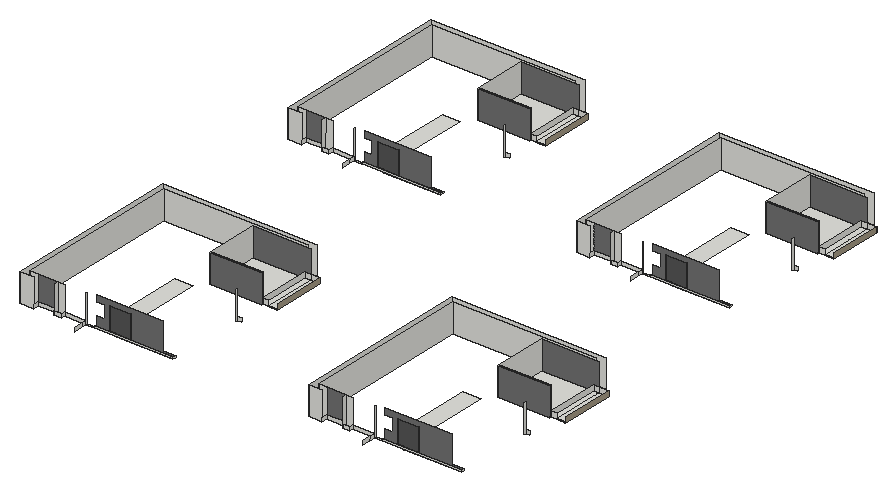
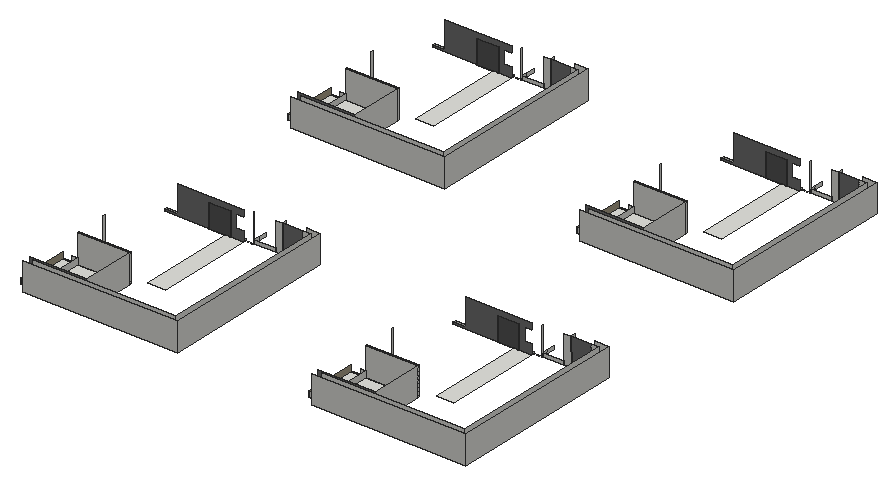
# SketchUp Ruby script. Lengths in inches.
U = 1.inch
M = Sketchup.active_model
def pt(a) = Geom::Point3d.new(a.map { |v| v * U })
def face(e, loops, mat)
  f = e.add_face(loops[0].map { |a| pt(a) })
  loops[1..].each { |l| e.add_face(l.map { |a| pt(a) }).erase! }
  f.material = f.back_material = mat if mat
  f
end
# faces: each face lists its corners as indices into pts; further lists are holes
def faces(e, pts, list, mat = nil) = list.each { |f| face(e, (f[0].is_a?(Array) ? f : [f]).map { |l| l.map { |i| pts[i] } }, mat) }
# xy, xz, yz: faces in a plane at the given z, y or x. An outline is a flat list of corners, or four numbers for a rectangle; further outlines are holes
def ring(l) = l.size == 4 ? [[l[0], l[1]], [l[2], l[1]], [l[2], l[3]], [l[0], l[3]]] : l.each_slice(2).to_a
def flat(e, list, mat, &to3) = list.each { |f| face(e, (f[0].is_a?(Array) ? f : [f]).map { |l| ring(l).map { |u, v| to3.(u, v) } }, mat) }
def xy(e, z, list, mat = nil) = flat(e, list, mat) { |x, y| [x, y, z] }
def xz(e, y, list, mat = nil) = flat(e, list, mat) { |x, z| [x, y, z] }
def yz(e, x, list, mat = nil) = flat(e, list, mat) { |y, z| [x, y, z] }
def lines(e, pts, list) = list.each { |a, b| e.add_line(pt(pts[a]), pt(pts[b])) }
# prism: a flat outline (further loops are holes) pulled along v
def prism(e, loops, v, mat = nil)
  f = face(e, loops, mat); d = Geom::Vector3d.new(v.map { |x| x * U })
  f.pushpull(f.normal.samedirection?(d) ? d.length : -d.length)
end
def box(e, o, s, mat = nil) = prism(e, [[o, [o[0] + s[0], o[1], o[2]], [o[0] + s[0], o[1] + s[1], o[2]], [o[0], o[1] + s[1], o[2]]]], [0, 0, s[2]], mat)
def at(x, y, z, deg = 0) = Geom::Transformation.translation(pt([x, y, z])) * Geom::Transformation.rotation(ORIGIN, Z_AXIS, deg.degrees)
def axes(o, x, y, z) = Geom::Transformation.new([*x, 0, *y, 0, *z, 0, *pt(o).to_a, 1])
def part(name) = M.definitions.add(name)
# library, detail: a bought-in or finely detailed component or shape, given as its bounding box
def library(name, o, s) = part(name).tap { |d| box(d.entities, o, s) }
def detail(e, o, s) = box(e.add_group.entities, o, s)
def put(e, d, t, mat = nil) = e.add_instance(d, t).tap { |i| i.material = mat if mat }
def group(e, t, mat = nil) = e.add_group.tap { |g| g.transformation = t; g.material = mat if mat }.entities
root = M.entities
M.materials.add("[Color M05]").color = [114, 114, 114]
M.materials.add("[Color M06]").color = [86, 86, 86]
M.materials.add("[Concrete Tile]").color = [165, 155, 133]
M.materials.add("[Granite Brown]").color = [89, 59, 61]
xy(root,510,[[523.04,1822.9375,557.4,1827.4375],[648.79,1822.9375,650.48,1827.4375],[650.48,1822.9375,890.875,1822.9375,890.875,1835.1875,701.59,1835.1875,701.59,1837.0625,650.48,1837.0625],[1741.23,1822.9375,1775.59,1827.4375],[1866.98,1822.9375,1868.66,1827.4375],
  [1868.66,1822.9375,2109.0625,1822.9375,2109.0625,1835.1875,1919.77,1835.1875,1919.77,1837.0625,1868.66,1837.0625],[557.88,1827.4375,632.49,1829.625],[632.49,1827.4375,648.79,1837.0625],[648.79,1827.4375,650.48,1837.0625],[1776.07,1827.4375,1850.67,1829.625],
  [1850.67,1827.4375,1866.98,1837.0625],[1866.98,1827.4375,1868.66,1837.0625],[557.88,1829.625,632.49,1835.1875],[1776.07,1829.625,1850.67,1835.1875],[557.4,1835.1875,632.49,2246.6875],
  [1775.59,1835.1875,1850.67,2246.6875],[671.875,2290,890.875,2295.875],[1890.0625,2290,2109.0625,2295.875],[671.875,2295.875,890.875,2518.89],[890.875,2295.875,913.875,2518.89],
  [913.875,2295.875,954.6875,2518.89],[1890.0625,2295.875,2109.0625,2518.89],[2109.0625,2295.875,2132.0625,2518.89],[2132.0625,2295.875,2172.875,2518.89],[523.04,3237.625,557.4,3242.125],
  [648.79,3237.625,650.48,3242.125],[650.48,3237.625,890.875,3237.625,890.875,3249.875,701.59,3249.875,701.59,3251.75,650.48,3251.75],[1741.23,3237.625,1775.59,3242.125],[1866.98,3237.625,1868.66,3242.125],[1868.66,3237.625,2109.0625,3237.625,2109.0625,3249.875,1919.77,3249.875,1919.77,3251.75,1868.66,3251.75],
  [557.88,3242.125,632.49,3244.3125],[632.49,3242.125,648.79,3251.75],[648.79,3242.125,650.48,3251.75],[1776.07,3242.125,1850.67,3244.3125],[1850.67,3242.125,1866.98,3251.75],
  [1866.98,3242.125,1868.66,3251.75],[557.88,3244.3125,632.49,3249.875],[1776.07,3244.3125,1850.67,3249.875],[557.4,3249.875,632.49,3661.375],[1775.59,3249.875,1850.67,3661.375],
  [671.875,3704.6875,890.875,3710.5625],[1890.0625,3704.6875,2109.0625,3710.5625],[671.875,3710.5625,890.875,3933.57],[890.875,3710.5625,913.875,3933.57],[913.875,3710.5625,954.6875,3933.57],
  [1890.0625,3710.5625,2109.0625,3933.57],[2109.0625,3710.5625,2132.0625,3933.57],[2132.0625,3710.5625,2172.875,3933.57]])
xy(root,510,[[557.4,1822.9375,557.88,1827.4375],[1775.59,1822.9375,1776.07,1827.4375],[557.4,1827.4375,557.88,1829.625],[1775.59,1827.4375,1776.07,1829.625],[557.4,1829.625,557.88,1835.1875],
  [1775.59,1829.625,1776.07,1835.1875],[557.4,3237.625,557.88,3242.125],[1775.59,3237.625,1776.07,3242.125],[557.4,3242.125,557.88,3244.3125],[1775.59,3242.125,1776.07,3244.3125],
  [557.4,3244.3125,557.88,3249.875],[1775.59,3244.3125,1776.07,3249.875]],"[Granite Brown]")
xy(root,510.3125,[[611.65,1835.1875,632.49,1837.0625],[1829.84,1835.1875,1850.67,1837.0625],[611.65,3249.875,632.49,3251.75],[1829.84,3249.875,1850.67,3251.75]])
xz(root,1799.9375,[[262.875,510,319.53,630],[1481.0625,510,1537.72,630]])
xz(root,1806.5625,[[401.17,510,401.17,525.4375,401.25,525.4375],[401.17,510,431.33,510,431.33,525.4375,401.25,525.4375],[1619.36,510,1619.36,525.4375,1619.4375,525.4375],[1619.36,510,1649.52,510,1649.52,525.4375,1619.4375,525.4375]])
xz(root,1822.9375,[[285.875,510,319.53,630],[319.53,510,401.17,525.4375],[401.17,510,401.77,630,431.33,630,431.33,510],[431.33,510,523.04,525.4375],[557.88,510,890.875,516.375],
  [1504.0625,510,1537.72,630],[1537.72,510,1619.36,525.4375],[1619.36,510,1619.96,630,1649.52,630,1649.52,510],[1649.52,510,1741.23,525.4375],[1776.07,510,2109.0625,516.375]])
xz(root,1822.9375,[[401.17,510,401.77,630,319.53,630,319.53,525.4375,401.17,525.4375],[1619.36,510,1619.96,630,1537.72,630,1537.72,525.4375,1619.36,525.4375]],"[Color M05]")
xz(root,1835.1875,[[611.65,509.5625,632.49,510],[1829.84,509.5625,1850.67,510],[611.65,510,632.49,510.3125],[1829.84,510,1850.67,510.3125]])
xz(root,1835.1875,[[557.88,510,611.65,510,611.65,608.125,701.59,608.125,701.59,510,890.875,510,890.875,517.25,838.125,517.25,838.125,630,557.88,630,557.88,603.53,589.71,603.53,589.71,551.24,557.88,551.24],[1776.07,510,1829.84,510,1829.84,608.125,1919.77,608.125,1919.77,510,2109.0625,510,2109.0625,517.25,2056.3125,517.25,2056.3125,630,1776.07,630,1776.07,603.53,1807.9,603.53,1807.9,551.24,1776.07,551.24]],"[Color M05]")
xz(root,1837.0625,[[632.49,510,701.59,510,701.59,608.125,611.65,608.125,611.65,510.3125,632.49,510.3125],[1850.67,510,1919.77,510,1919.77,608.125,1829.84,608.125,1829.84,510.3125,1850.67,510.3125]],"[Color M06]")
xz(root,2156.01,[[894.3125,510,913.875,527.36],[2112.5,510,2132.0625,527.36]])
xz(root,2290,[[671.875,510,890.875,630],[1890.0625,510,2109.0625,630]],"[Color M05]")
xz(root,2295.875,[[671.875,510,890.875,630],[890.875,510,913.875,534.0625],[913.875,510,930.75,511.75],[930.75,510,954.6875,511.75],[1890.0625,510,2109.0625,630],
  [2109.0625,510,2132.0625,534.0625],[2132.0625,510,2148.9375,511.75],[2148.9375,510,2172.875,511.75]])
xz(root,2518.89,[[890.875,510,913.875,534.0625],[913.875,510,954.6875,534.0625],[2109.0625,510,2132.0625,534.0625],[2132.0625,510,2172.875,534.0625]])
xz(root,2518.89,[[671.875,510,890.875,510,890.875,534.0625,913.875,534.0625,913.875,630,671.875,630],[1890.0625,510,2109.0625,510,2109.0625,534.0625,2132.0625,534.0625,2132.0625,630,1890.0625,630]],"[Color M05]")
xz(root,2531.375,[[285.875,510,890.875,630],[1504.0625,510,2109.0625,630]])
xz(root,2554.375,[[262.875,510,913.875,630],[1481.0625,510,2132.0625,630]])
xz(root,3214.625,[[262.875,510,319.53,630],[1481.0625,510,1537.72,630]])
xz(root,3221.25,[[401.17,510,401.17,525.4375,401.25,525.4375],[401.17,510,431.33,510,431.33,525.4375,401.25,525.4375],[1619.36,510,1619.36,525.4375,1619.4375,525.4375],[1619.36,510,1649.52,510,1649.52,525.4375,1619.4375,525.4375]])
xz(root,3237.625,[[285.875,510,319.53,630],[319.53,510,401.17,525.4375],[401.17,510,401.77,630,431.33,630,431.33,510],[431.33,510,523.04,525.4375],[557.88,510,890.875,516.375],
  [1504.0625,510,1537.72,630],[1537.72,510,1619.36,525.4375],[1619.36,510,1619.96,630,1649.52,630,1649.52,510],[1649.52,510,1741.23,525.4375],[1776.07,510,2109.0625,516.375]])
xz(root,3237.625,[[401.17,510,401.77,630,319.53,630,319.53,525.4375,401.17,525.4375],[1619.36,510,1619.96,630,1537.72,630,1537.72,525.4375,1619.36,525.4375]],"[Color M05]")
xz(root,3249.875,[[611.65,509.5625,632.49,510],[1829.84,509.5625,1850.67,510],[611.65,510,632.49,510.3125],[1829.84,510,1850.67,510.3125]])
xz(root,3249.875,[[557.88,510,611.65,510,611.65,608.125,701.59,608.125,701.59,510,890.875,510,890.875,517.25,838.125,517.25,838.125,630,557.88,630,557.88,603.53,589.71,603.53,589.71,551.24,557.88,551.24],[1776.07,510,1829.84,510,1829.84,608.125,1919.77,608.125,1919.77,510,2109.0625,510,2109.0625,517.25,2056.3125,517.25,2056.3125,630,1776.07,630,1776.07,603.53,1807.9,603.53,1807.9,551.24,1776.07,551.24]],"[Color M05]")
xz(root,3251.75,[[632.49,510,701.59,510,701.59,608.125,611.65,608.125,611.65,510.3125,632.49,510.3125],[1850.67,510,1919.77,510,1919.77,608.125,1829.84,608.125,1829.84,510.3125,1850.67,510.3125]],"[Color M06]")
xz(root,3570.7,[[894.3125,510,913.875,527.36],[2112.5,510,2132.0625,527.36]])
xz(root,3704.6875,[[671.875,510,890.875,630],[1890.0625,510,2109.0625,630]],"[Color M05]")
xz(root,3710.5625,[[671.875,510,890.875,630],[890.875,510,913.875,534.0625],[913.875,510,930.75,511.75],[930.75,510,954.6875,511.75],[1890.0625,510,2109.0625,630],
  [2109.0625,510,2132.0625,534.0625],[2132.0625,510,2148.9375,511.75],[2148.9375,510,2172.875,511.75]])
xz(root,3933.57,[[890.875,510,913.875,534.0625],[913.875,510,954.6875,534.0625],[2109.0625,510,2132.0625,534.0625],[2132.0625,510,2172.875,534.0625]])
xz(root,3933.57,[[671.875,510,890.875,510,890.875,534.0625,913.875,534.0625,913.875,630,671.875,630],[1890.0625,510,2109.0625,510,2109.0625,534.0625,2132.0625,534.0625,2132.0625,630,1890.0625,630]],"[Color M05]")
xz(root,3946.0625,[[285.875,510,890.875,630],[1504.0625,510,2109.0625,630]])
xz(root,3969.0625,[[262.875,510,913.875,630],[1481.0625,510,2132.0625,630]])
yz(root,262.875,[[1799.9375,510,2554.375,630],[3214.625,510,3969.0625,630]])
yz(root,285.875,[[1822.9375,510,2531.375,630],[3237.625,510,3946.0625,630]])
yz(root,319.53,[[1799.9375,510,1822.9375,525.4375],[3214.625,510,3237.625,525.4375]])
yz(root,401.17,[[1806.5625,510,1822.9375,525.4375],[3221.25,510,3237.625,525.4375]])
yz(root,431.33,[[1806.5625,510,1822.9375,525.4375],[3221.25,510,3237.625,525.4375]])
yz(root,523.04,[[1763.25,510,1799.9375,525.4375],[1799.9375,510,1822.9375,525.4375],[1822.9375,510,1827.4375,630],[3177.9375,510,3214.625,525.4375],[3214.625,510,3237.625,525.4375],
  [3237.625,510,3242.125,630]])
yz(root,611.65,[[1835.1875,510.3125,1837.0625,608.125],[3249.875,510.3125,3251.75,608.125]])
yz(root,632.49,[[1835.1875,510,1837.0625,510.3125],[3249.875,510,3251.75,510.3125]])
yz(root,671.875,[[2290,510,2295.875,630],[2295.875,510,2518.89,630],[3704.6875,510,3710.5625,630],[3710.5625,510,3933.57,630]])
yz(root,701.59,[[1835.1875,510,1837.0625,608.125],[3249.875,510,3251.75,608.125]])
yz(root,890.875,[[1822.9375,510,1835.1875,516.375],[2290,510,2295.875,511.75],[2295.875,510,2518.89,534.0625],[3237.625,510,3249.875,516.375],[3704.6875,510,3710.5625,511.75],
  [3710.5625,510,3933.57,534.0625]])
yz(root,894.3125,[[2148.83,510,2156.01,630],[3563.51,510,3570.7,630]])
yz(root,954.6875,[[2295.875,510,2518.89,534.0625],[3710.5625,510,3933.57,534.0625]],"[Concrete Tile]")
yz(root,1481.0625,[[1799.9375,510,2554.375,630],[3214.625,510,3969.0625,630]])
yz(root,1504.0625,[[1822.9375,510,2531.375,630],[3237.625,510,3946.0625,630]])
yz(root,1537.72,[[1799.9375,510,1822.9375,525.4375],[3214.625,510,3237.625,525.4375]])
yz(root,1619.36,[[1806.5625,510,1822.9375,525.4375],[3221.25,510,3237.625,525.4375]])
yz(root,1649.52,[[1806.5625,510,1822.9375,525.4375],[3221.25,510,3237.625,525.4375]])
yz(root,1741.23,[[1763.25,510,1799.9375,525.4375],[1799.9375,510,1822.9375,525.4375],[1822.9375,510,1827.4375,630],[3177.9375,510,3214.625,525.4375],[3214.625,510,3237.625,525.4375],
  [3237.625,510,3242.125,630]])
yz(root,1829.84,[[1835.1875,510.3125,1837.0625,608.125],[3249.875,510.3125,3251.75,608.125]])
yz(root,1850.67,[[1835.1875,510,1837.0625,510.3125],[3249.875,510,3251.75,510.3125]])
yz(root,1890.0625,[[2290,510,2295.875,630],[2295.875,510,2518.89,630],[3704.6875,510,3710.5625,630],[3710.5625,510,3933.57,630]])
yz(root,1919.77,[[1835.1875,510,1837.0625,608.125],[3249.875,510,3251.75,608.125]])
yz(root,2109.0625,[[1822.9375,510,1835.1875,516.375],[2290,510,2295.875,511.75],[2295.875,510,2518.89,534.0625],[3237.625,510,3249.875,516.375],[3704.6875,510,3710.5625,511.75],
  [3710.5625,510,3933.57,534.0625]])
yz(root,2112.5,[[2148.83,510,2156.01,630],[3563.51,510,3570.7,630]])
yz(root,2172.875,[[2295.875,510,2518.89,534.0625],[3710.5625,510,3933.57,534.0625]],"[Concrete Tile]")
p = [[401.17,1822.9375,510],[401.17,1806.5625,510],[401.25,1806.5625,525.4375],[401.77,1806.5625,630],[401.77,1822.9375,630],[1619.36,1822.9375,510],
  [1619.36,1806.5625,510],[1619.4375,1806.5625,525.4375],[1619.96,1806.5625,630],[1619.96,1822.9375,630],[401.17,3237.625,510],[401.17,3221.25,510],
  [401.25,3221.25,525.4375],[401.77,3221.25,630],[401.77,3237.625,630],[1619.36,3237.625,510],[1619.36,3221.25,510],[1619.4375,3221.25,525.4375],
  [1619.96,3221.25,630],[1619.96,3237.625,630],[1619.36,1799.9375,510],[1649.52,1799.9375,510],[1649.52,1806.5625,510],[1829.84,1835.1875,507.5],
  [1850.67,1835.1875,507.5],[1919.77,1835.1875,507.5],[1919.77,1835.1875,509.5625],[1919.77,1835.1875,510],[1829.84,1835.1875,509.5625],[1741.23,1778.3125,510],
  [1741.23,1778.3125,525.4375],[431.33,1799.9375,510],[431.33,1806.5625,510],[401.17,1799.9375,510],[632.49,1835.1875,507.5],[701.59,1835.1875,507.5],
  [701.59,1835.1875,509.5625],[611.65,1835.1875,507.5],[611.65,1835.1875,509.5625],[701.59,1835.1875,510],[523.04,1778.3125,510],[523.04,1778.3125,525.4375],
  [1741.23,3193,510],[1741.23,3193,525.4375],[1649.52,3214.625,510],[1649.52,3221.25,510],[1619.36,3214.625,510],[1850.67,3249.875,507.5],
  [1919.77,3249.875,507.5],[1829.84,3249.875,507.5],[1919.77,3249.875,509.5625],[1829.84,3249.875,509.5625],[1919.77,3249.875,510],[431.33,3214.625,510],
  [431.33,3221.25,510],[401.17,3214.625,510],[632.49,3249.875,507.5],[701.59,3249.875,507.5],[611.65,3249.875,507.5],[701.59,3249.875,509.5625],
  [611.65,3249.875,509.5625],[701.59,3249.875,510],[523.04,3193,510],[523.04,3193,525.4375]]
faces(root,p,[[0,1,2,3,4],[5,6,7,8,9],[10,11,12,13,14],[15,16,17,18,19]])
lines(root,p,[[20,6],[21,22],[23,24],[25,26],[24,25],[26,27],[28,23],[29,30],[31,32],[33,1],[34,35],[35,36],
  [37,34],[38,37],[36,39],[40,41],[42,43],[44,45],[46,16],[47,48],[49,47],[48,50],[51,49],[50,52],
  [53,54],[55,11],[56,57],[58,56],[57,59],[60,58],[59,61],[62,63]])
